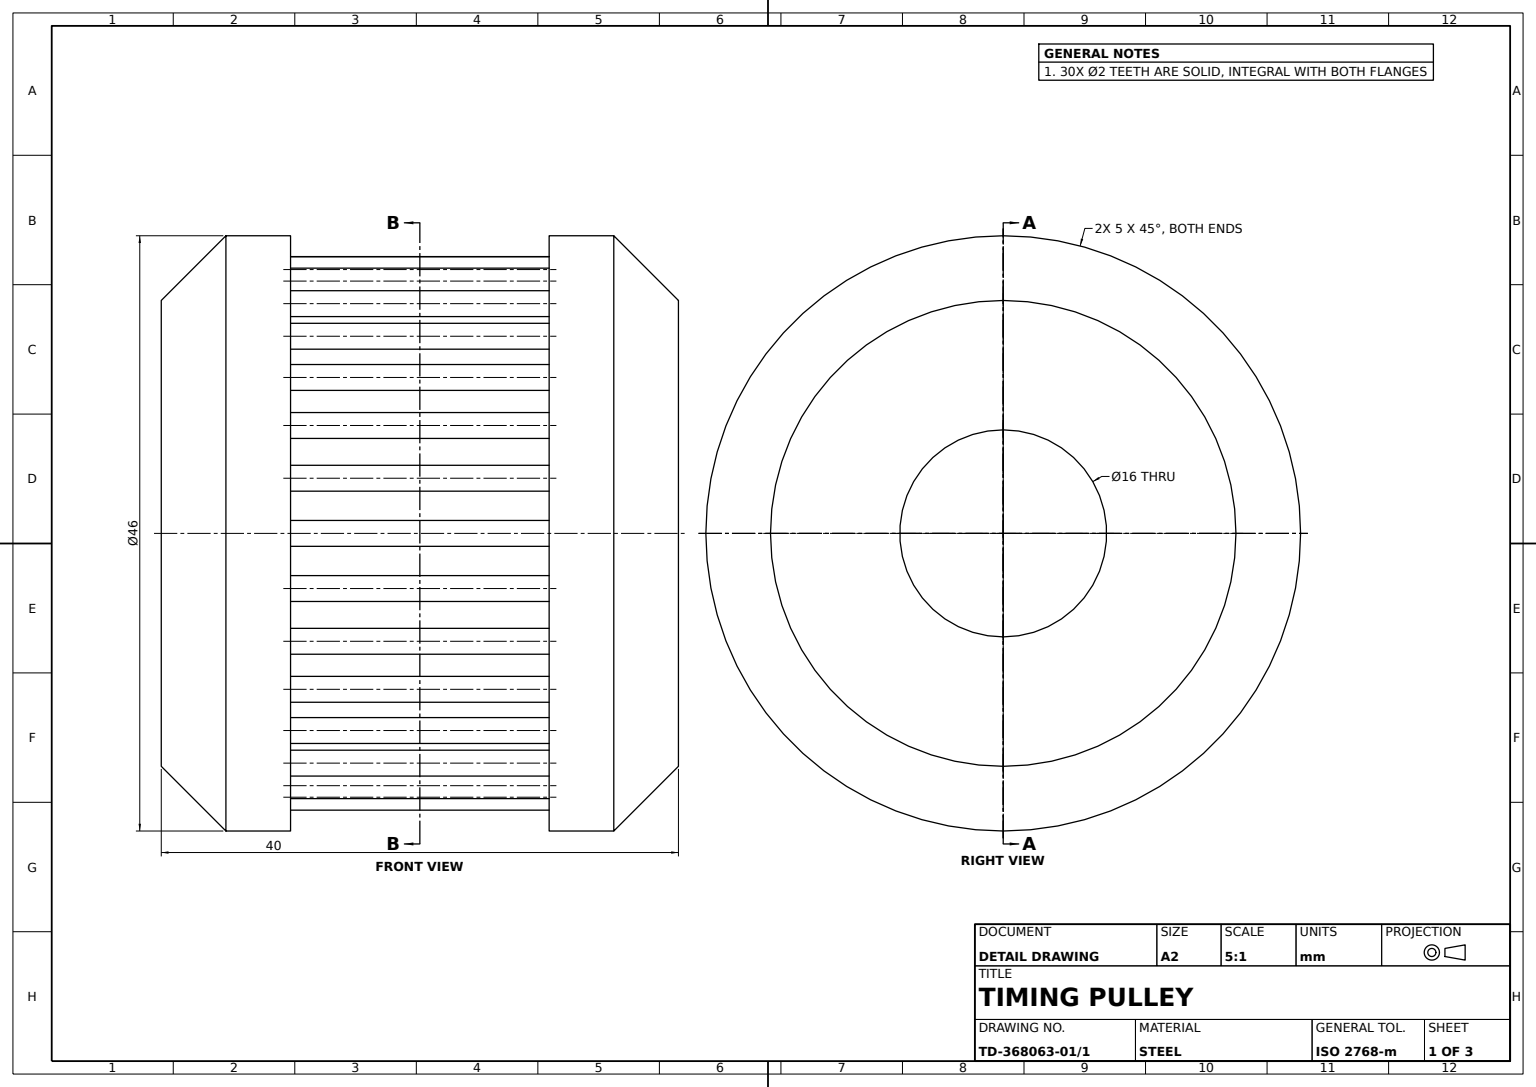
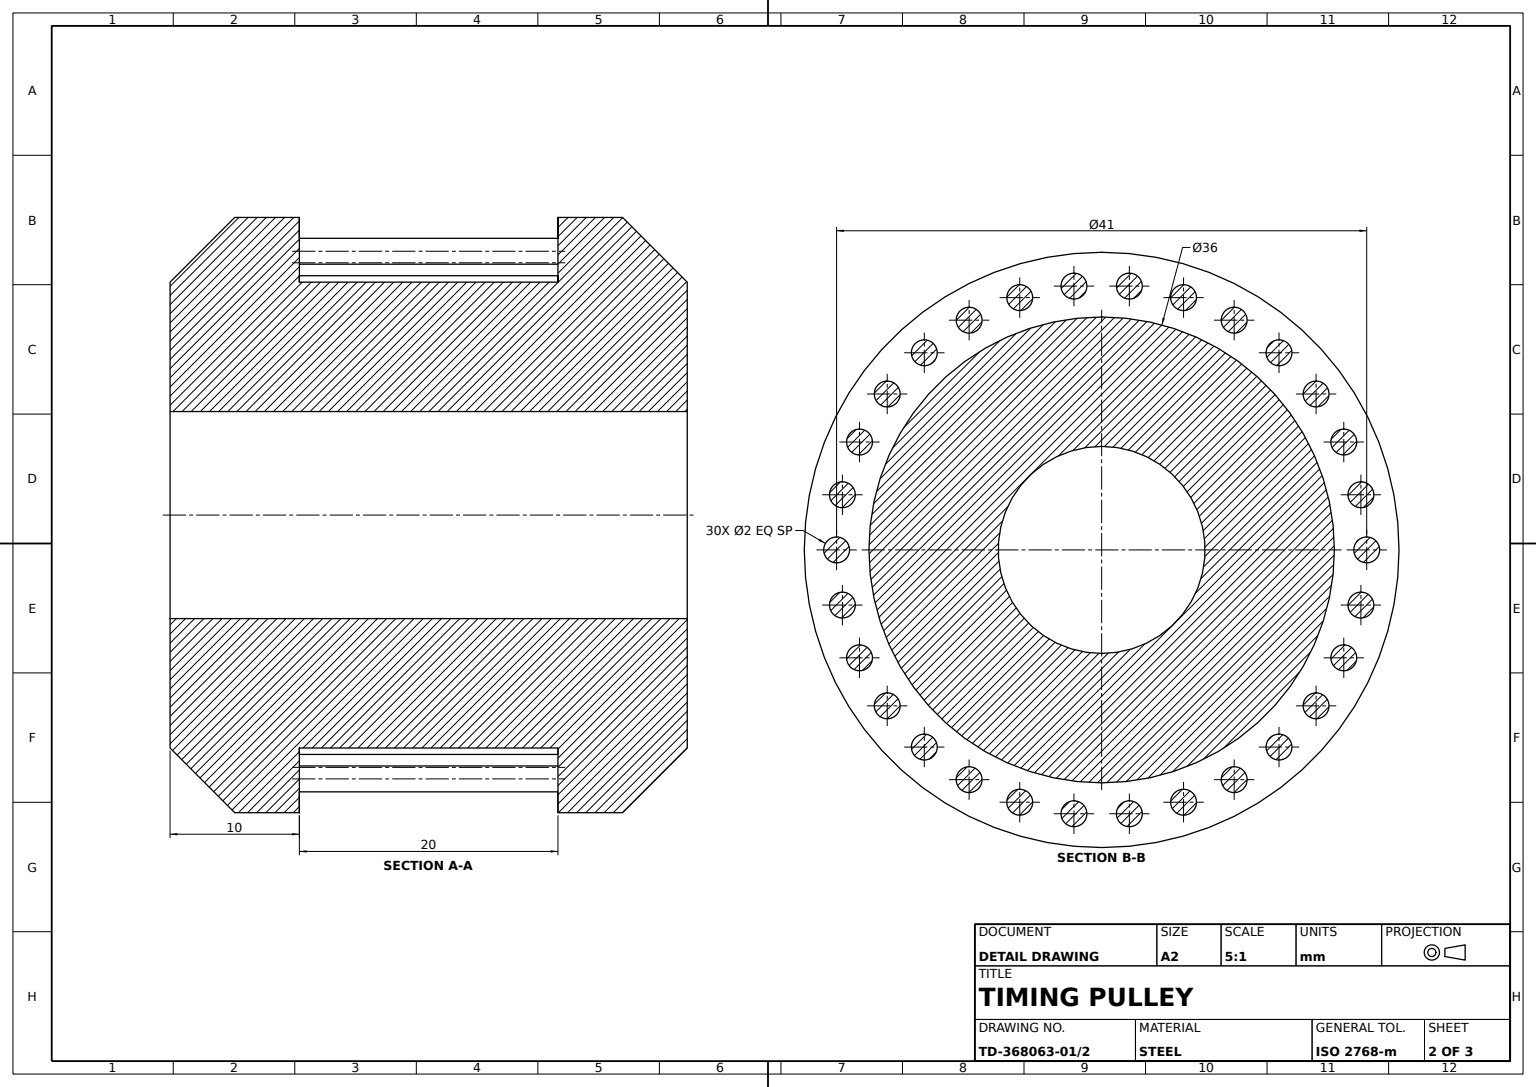
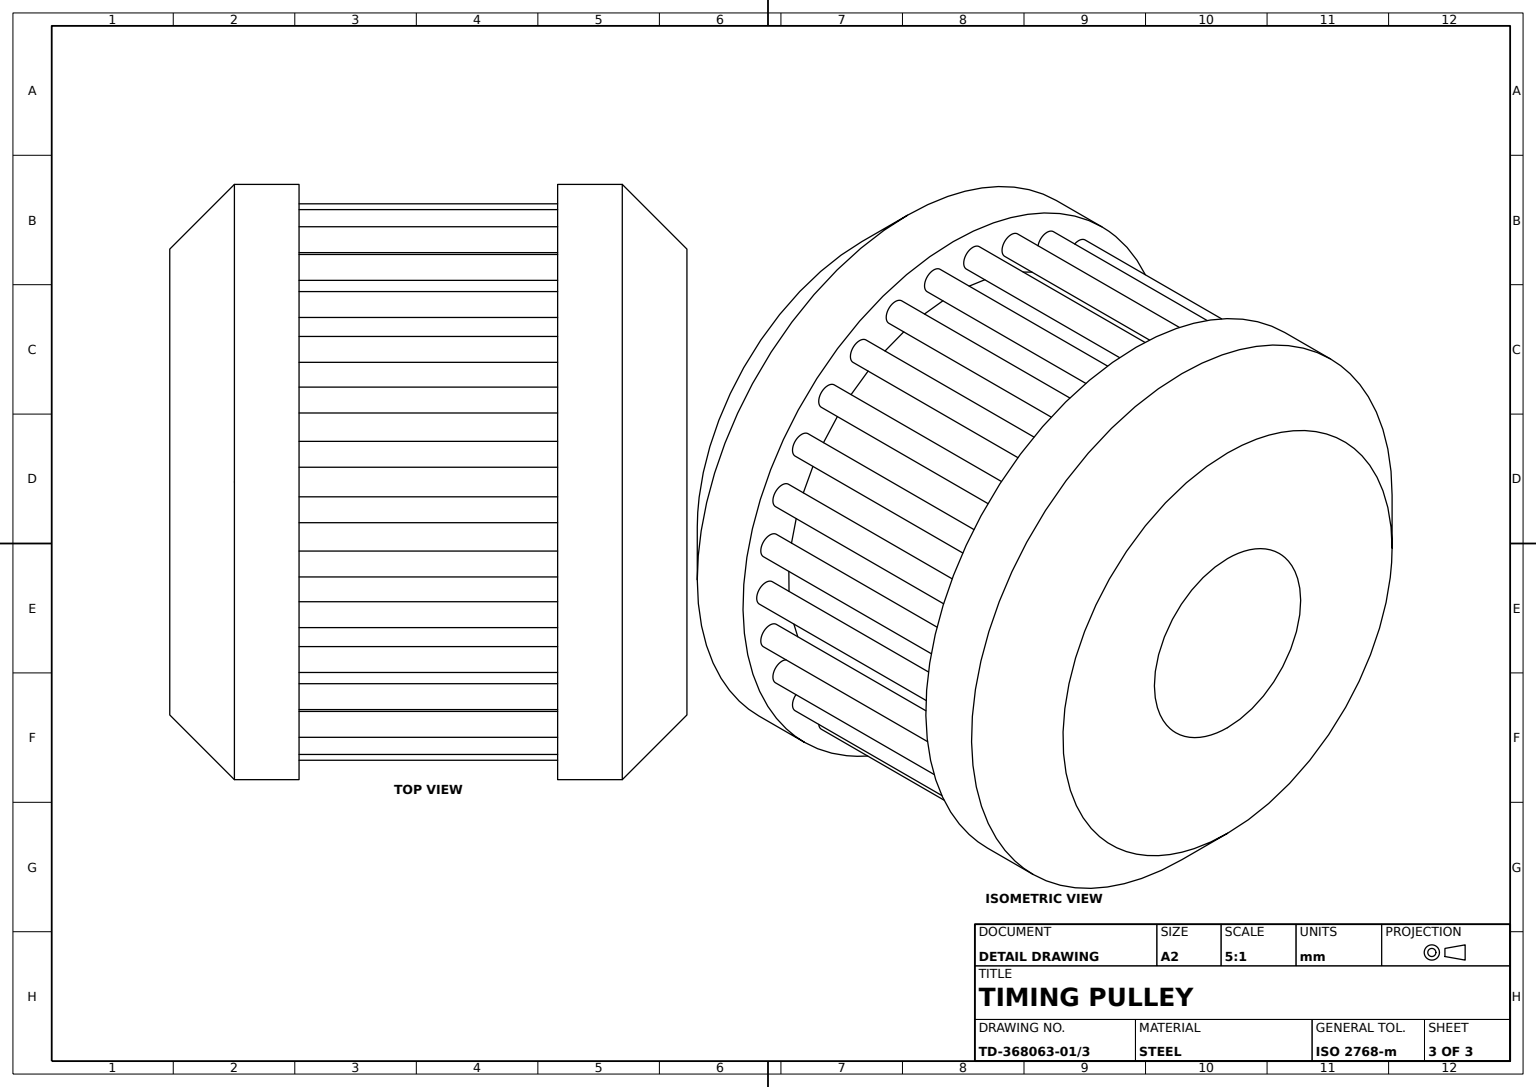
solid
v1 (-1,30,20.5)
v2 (1,30,20.5)
e1 v1 v2 CIRCLE(AX(P(0,30,20.5),D(0,-1,0),D(-1,0,0)),1)
v3 (1,10,20.5)
e2 v3 v2 LINE
v4 (-1,10,20.5)
e3 v3 v4 CIRCLE(AX(P(0,10,20.5),D(0,1,0),D(1,0,0)),1)
e4 v4 v1 LINE
face CYL(AX(P(0,10,20.5),D(0,1,0),D(-1,0,0)),1) [e1 -e2 e3 e4]
v5 (18.496659,30,-6.334848)
v6 (20.496659,30,-6.334848)
e5 v5 v6 CIRCLE(AX(P(19.496659,30,-6.334848),D(0,-1,0),D(-1,0,0)),1)
v7 (20.496659,10,-6.334848)
e6 v7 v6 LINE
v8 (18.496659,10,-6.334848)
e7 v7 v8 CIRCLE(AX(P(19.496659,10,-6.334848),D(0,1,0),D(1,0,0)),1)
e8 v8 v5 LINE
face CYL(AX(P(19.496659,10,-6.334848),D(0,1,0),D(-1,0,0)),1) [e5 -e6 e7 e8]
v9 (-18,30,0)
v10 (18,30,0)
e9 v9 v10 CIRCLE(AX(P(0,30,0),D(0,1,0),D(-1,0,0)),18)
v11 (-18,10,0)
e10 v11 v9 LINE
v12 (18,10,0)
e11 v11 v12 CIRCLE(AX(P(0,10,0),D(0,1,0),D(-1,0,0)),18)
e12 v12 v10 LINE
face CYL(AX(P(0,32.636364,0),D(0,1,0),D(-1,0,0)),18) [-e9 -e10 e11 e12]
v13 (19.387699,30,-2.142833)
v14 (21.387699,30,-2.142833)
e13 v13 v14 CIRCLE(AX(P(20.387699,30,-2.142833),D(0,-1,0),D(-1,0,0)),1)
v15 (21.387699,10,-2.142833)
e14 v15 v14 LINE
v16 (19.387699,10,-2.142833)
e15 v15 v16 CIRCLE(AX(P(20.387699,10,-2.142833),D(0,1,0),D(1,0,0)),1)
e16 v16 v13 LINE
face CYL(AX(P(20.387699,10,-2.142833),D(0,1,0),D(-1,0,0)),1) [e13 -e14 e15 e16]
v17 (23,30,0)
v18 (23,35,0)
e17 v17 v18 LINE
v19 (-23,35,0)
e18 v19 v18 CIRCLE(AX(P(0,35,0),D(0,1,0),D(-1,0,0)),23)
v20 (-23,30,0)
e19 v20 v19 LINE
e20 v20 v17 CIRCLE(AX(P(0,30,0),D(0,1,0),D(-1,0,0)),23)
face CYL(AX(P(0,32.636364,0),D(0,1,0),D(-1,0,0)),23) [e17 -e18 -e19 e20]
v21 (18,0,0)
v22 (-18,0,0)
e21 v21 v22 CIRCLE(AX(P(0,0,0),D(0,1,0),D(-1,0,0)),18)
v23 (-23,5,0)
e22 v22 v23 LINE
v24 (23,5,0)
e23 v24 v23 CIRCLE(AX(P(0,5,0),D(0,1,0),D(-1,0,0)),23)
e24 v21 v24 LINE
face CONE(AX(P(0,0,0),D(0,1,0),D(-1,0,0)),18,0.785398163) [e21 e22 -e23 -e24]
v25 (18,40,0)
e25 v25 v18 LINE
v26 (-18,40,0)
e26 v26 v25 CIRCLE(AX(P(0,40,0),D(0,1,0),D(-1,0,0)),18)
e27 v26 v19 LINE
face CONE(AX(P(0,35,0),D(0,-1,0),D(1,0,0)),23,0.785398163) [e18 -e25 -e26 e27]
v27 (-9.338101,30,18.727682)
v28 (-7.338101,30,18.727682)
e28 v27 v28 CIRCLE(AX(P(-8.338101,30,18.727682),D(0,-1,0),D(-1,0,0)),1)
v29 (-7.338101,10,18.727682)
e29 v29 v28 LINE
v30 (-9.338101,10,18.727682)
e30 v29 v30 CIRCLE(AX(P(-8.338101,10,18.727682),D(0,1,0),D(1,0,0)),1)
e31 v30 v27 LINE
face CYL(AX(P(-8.338101,10,18.727682),D(0,1,0),D(-1,0,0)),1) [e28 -e29 e30 e31]
v31 (-20.496659,10,6.334848)
v32 (-18.496659,10,6.334848)
e32 v31 v32 CIRCLE(AX(P(-19.496659,10,6.334848),D(0,1,0),D(1,0,0)),1)
v33 (-18.496659,30,6.334848)
e33 v32 v33 LINE
v34 (-20.496659,30,6.334848)
e34 v33 v34 CIRCLE(AX(P(-19.496659,30,6.334848),D(0,-1,0),D(-1,0,0)),1)
e35 v31 v34 LINE
face CYL(AX(P(-19.496659,10,6.334848),D(0,1,0),D(-1,0,0)),1) [e32 e33 e34 -e35]
v35 (14.234469,10,-13.717177)
v36 (16.234469,10,-13.717177)
e36 v35 v36 CIRCLE(AX(P(15.234469,10,-13.717177),D(0,1,0),D(1,0,0)),1)
v37 (16.234469,30,-13.717177)
e37 v36 v37 LINE
v38 (14.234469,30,-13.717177)
e38 v37 v38 CIRCLE(AX(P(15.234469,30,-13.717177),D(0,-1,0),D(-1,0,0)),1)
e39 v35 v38 LINE
face CYL(AX(P(15.234469,10,-13.717177),D(0,1,0),D(-1,0,0)),1) [e36 e37 e38 -e39]
e40 v12 v11 CIRCLE(AX(P(0,10,0),D(0,1,0),D(-1,0,0)),18)
e41 v10 v9 CIRCLE(AX(P(0,30,0),D(0,1,0),D(-1,0,0)),18)
face CYL(AX(P(0,32.636364,0),D(0,1,0),D(-1,0,0)),18) [e40 e10 -e41 -e12]
v39 (21.387699,10,2.142833)
v40 (19.387699,10,2.142833)
e42 v39 v40 CIRCLE(AX(P(20.387699,10,2.142833),D(0,1,0),D(1,0,0)),1)
v41 (19.387699,30,2.142833)
e43 v40 v41 LINE
v42 (21.387699,30,2.142833)
e44 v41 v42 CIRCLE(AX(P(20.387699,30,2.142833),D(0,-1,0),D(-1,0,0)),1)
e45 v39 v42 LINE
face CYL(AX(P(20.387699,10,2.142833),D(0,1,0),D(-1,0,0)),1) [e42 e43 e44 -e45]
v43 (20.496659,10,6.334848)
v44 (20.496659,30,6.334848)
e46 v43 v44 LINE
v45 (18.496659,10,6.334848)
e47 v43 v45 CIRCLE(AX(P(19.496659,10,6.334848),D(0,1,0),D(1,0,0)),1)
v46 (18.496659,30,6.334848)
e48 v45 v46 LINE
e49 v46 v44 CIRCLE(AX(P(19.496659,30,6.334848),D(0,-1,0),D(-1,0,0)),1)
face CYL(AX(P(19.496659,10,6.334848),D(0,1,0),D(-1,0,0)),1) [-e46 e47 e48 e49]
v47 (9.338101,10,-18.727682)
v48 (9.338101,30,-18.727682)
e50 v47 v48 LINE
v49 (7.338101,30,-18.727682)
e51 v48 v49 CIRCLE(AX(P(8.338101,30,-18.727682),D(0,-1,0),D(-1,0,0)),1)
v50 (7.338101,10,-18.727682)
e52 v50 v49 LINE
e53 v50 v47 CIRCLE(AX(P(8.338101,10,-18.727682),D(0,1,0),D(1,0,0)),1)
face CYL(AX(P(8.338101,10,-18.727682),D(0,1,0),D(-1,0,0)),1) [e50 e51 -e52 e53]
e54 v18 v19 CIRCLE(AX(P(0,35,0),D(0,1,0),D(-1,0,0)),23)
e55 v25 v26 CIRCLE(AX(P(0,40,0),D(0,1,0),D(-1,0,0)),18)
face CONE(AX(P(0,35,0),D(0,-1,0),D(1,0,0)),23,0.785398163) [e54 -e27 -e55 e25]
e56 v40 v39 CIRCLE(AX(P(20.387699,10,2.142833),D(0,1,0),D(1,0,0)),1)
e57 v42 v41 CIRCLE(AX(P(20.387699,30,2.142833),D(0,-1,0),D(-1,0,0)),1)
face CYL(AX(P(20.387699,10,2.142833),D(0,1,0),D(-1,0,0)),1) [-e43 e56 e45 e57]
v51 (-23,10,0)
e58 v23 v51 LINE
e59 v23 v24 CIRCLE(AX(P(0,5,0),D(0,1,0),D(-1,0,0)),23)
v52 (23,10,0)
e60 v24 v52 LINE
e61 v51 v52 CIRCLE(AX(P(0,10,0),D(0,1,0),D(-1,0,0)),23)
face CYL(AX(P(0,32.636364,0),D(0,1,0),D(-1,0,0)),23) [-e58 e59 e60 -e61]
e62 v32 v31 CIRCLE(AX(P(-19.496659,10,6.334848),D(0,1,0),D(1,0,0)),1)
e63 v34 v33 CIRCLE(AX(P(-19.496659,30,6.334848),D(0,-1,0),D(-1,0,0)),1)
face CYL(AX(P(-19.496659,10,6.334848),D(0,1,0),D(-1,0,0)),1) [e62 e35 e63 -e33]
v53 (-16.753521,10,10.25)
v54 (-18.753521,10,10.25)
e64 v53 v54 CIRCLE(AX(P(-17.753521,10,10.25),D(0,1,0),D(1,0,0)),1)
v55 (-18.753521,30,10.25)
e65 v54 v55 LINE
v56 (-16.753521,30,10.25)
e66 v55 v56 CIRCLE(AX(P(-17.753521,30,10.25),D(0,-1,0),D(-1,0,0)),1)
e67 v53 v56 LINE
face CYL(AX(P(-17.753521,10,10.25),D(0,1,0),D(-1,0,0)),1) [e64 e65 e66 -e67]
v57 (-19.387699,30,2.142833)
v58 (-21.387699,30,2.142833)
e68 v57 v58 CIRCLE(AX(P(-20.387699,30,2.142833),D(0,-1,0),D(-1,0,0)),1)
v59 (-21.387699,10,2.142833)
e69 v59 v58 LINE
v60 (-19.387699,10,2.142833)
e70 v59 v60 CIRCLE(AX(P(-20.387699,10,2.142833),D(0,1,0),D(1,0,0)),1)
e71 v60 v57 LINE
face CYL(AX(P(-20.387699,10,2.142833),D(0,1,0),D(-1,0,0)),1) [e68 -e69 e70 e71]
e72 v52 v51 CIRCLE(AX(P(0,10,0),D(0,1,0),D(-1,0,0)),23)
face CYL(AX(P(0,32.636364,0),D(0,1,0),D(-1,0,0)),23) [e58 -e72 -e60 e23]
v61 (5.26219,30,20.052026)
v62 (3.26219,30,20.052026)
e73 v61 v62 CIRCLE(AX(P(4.26219,30,20.052026),D(0,-1,0),D(-1,0,0)),1)
v63 (3.26219,10,20.052026)
e74 v63 v62 LINE
v64 (5.26219,10,20.052026)
e75 v63 v64 CIRCLE(AX(P(4.26219,10,20.052026),D(0,1,0),D(1,0,0)),1)
e76 v64 v61 LINE
face CYL(AX(P(4.26219,10,20.052026),D(0,1,0),D(-1,0,0)),1) [e73 -e74 e75 e76]
v65 (1,10,-20.5)
v66 (-1,10,-20.5)
e77 v65 v66 CIRCLE(AX(P(0,10,-20.5),D(0,1,0),D(1,0,0)),1)
v67 (-1,30,-20.5)
e78 v66 v67 LINE
v68 (1,30,-20.5)
e79 v67 v68 CIRCLE(AX(P(0,30,-20.5),D(0,-1,0),D(-1,0,0)),1)
e80 v65 v68 LINE
face CYL(AX(P(0,10,-20.5),D(0,1,0),D(-1,0,0)),1) [e77 e78 e79 -e80]
v69 (-8,0,0)
v70 (8,0,0)
e81 v69 v70 CIRCLE(AX(P(0,0,0),D(0,1,0),D(-1,0,0)),8)
v71 (-8,40,0)
e82 v69 v71 LINE
v72 (8,40,0)
e83 v71 v72 CIRCLE(AX(P(0,40,0),D(0,1,0),D(-1,0,0)),8)
e84 v70 v72 LINE
face CYL(AX(P(0,32.636364,0),D(0,1,0),D(-1,0,0)),8) rev [-e81 e82 e83 -e84]
v73 (18.753521,10,10.25)
v74 (18.753521,30,10.25)
e85 v73 v74 LINE
v75 (16.753521,10,10.25)
e86 v73 v75 CIRCLE(AX(P(17.753521,10,10.25),D(0,1,0),D(1,0,0)),1)
v76 (16.753521,30,10.25)
e87 v75 v76 LINE
e88 v76 v74 CIRCLE(AX(P(17.753521,30,10.25),D(0,-1,0),D(-1,0,0)),1)
face CYL(AX(P(17.753521,10,10.25),D(0,1,0),D(-1,0,0)),1) [-e85 e86 e87 e88]
v77 (13.049598,10,-16.584848)
v78 (13.049598,30,-16.584848)
e89 v77 v78 LINE
v79 (11.049598,10,-16.584848)
e90 v77 v79 CIRCLE(AX(P(12.049598,10,-16.584848),D(0,1,0),D(1,0,0)),1)
v80 (11.049598,30,-16.584848)
e91 v79 v80 LINE
e92 v80 v78 CIRCLE(AX(P(12.049598,30,-16.584848),D(0,-1,0),D(-1,0,0)),1)
face CYL(AX(P(12.049598,10,-16.584848),D(0,1,0),D(-1,0,0)),1) [-e89 e90 e91 e92]
e93 v45 v43 CIRCLE(AX(P(19.496659,10,6.334848),D(0,1,0),D(1,0,0)),1)
e94 v44 v46 CIRCLE(AX(P(19.496659,30,6.334848),D(0,-1,0),D(-1,0,0)),1)
face CYL(AX(P(19.496659,10,6.334848),D(0,1,0),D(-1,0,0)),1) [e93 e46 e94 -e48]
v81 (-16.753521,10,-10.25)
v82 (-16.753521,30,-10.25)
e95 v81 v82 LINE
v83 (-18.753521,10,-10.25)
e96 v81 v83 CIRCLE(AX(P(-17.753521,10,-10.25),D(0,1,0),D(1,0,0)),1)
v84 (-18.753521,30,-10.25)
e97 v83 v84 LINE
e98 v84 v82 CIRCLE(AX(P(-17.753521,30,-10.25),D(0,-1,0),D(-1,0,0)),1)
face CYL(AX(P(-17.753521,10,-10.25),D(0,1,0),D(-1,0,0)),1) [-e95 e96 e97 e98]
e99 v4 v3 CIRCLE(AX(P(0,10,20.5),D(0,1,0),D(1,0,0)),1)
e100 v2 v1 CIRCLE(AX(P(0,30,20.5),D(0,-1,0),D(-1,0,0)),1)
face CYL(AX(P(0,10,20.5),D(0,1,0),D(-1,0,0)),1) [-e4 e99 e2 e100]
v85 (-21.387699,10,-2.142833)
v86 (-21.387699,30,-2.142833)
e101 v85 v86 LINE
v87 (-19.387699,10,-2.142833)
e102 v85 v87 CIRCLE(AX(P(-20.387699,10,-2.142833),D(0,1,0),D(1,0,0)),1)
v88 (-19.387699,30,-2.142833)
e103 v87 v88 LINE
e104 v88 v86 CIRCLE(AX(P(-20.387699,30,-2.142833),D(0,-1,0),D(-1,0,0)),1)
face CYL(AX(P(-20.387699,10,-2.142833),D(0,1,0),D(-1,0,0)),1) [-e101 e102 e103 e104]
v89 (-5.26219,10,20.052026)
v90 (-5.26219,30,20.052026)
e105 v89 v90 LINE
v91 (-3.26219,30,20.052026)
e106 v90 v91 CIRCLE(AX(P(-4.26219,30,20.052026),D(0,-1,0),D(-1,0,0)),1)
v92 (-3.26219,10,20.052026)
e107 v92 v91 LINE
e108 v92 v89 CIRCLE(AX(P(-4.26219,10,20.052026),D(0,1,0),D(1,0,0)),1)
face CYL(AX(P(-4.26219,10,20.052026),D(0,1,0),D(-1,0,0)),1) [e105 e106 -e107 e108]
v93 (-5.26219,30,-20.052026)
v94 (-3.26219,30,-20.052026)
e109 v93 v94 CIRCLE(AX(P(-4.26219,30,-20.052026),D(0,-1,0),D(-1,0,0)),1)
e110 v94 v93 CIRCLE(AX(P(-4.26219,30,-20.052026),D(0,-1,0),D(-1,0,0)),1)
v95 (-16.234469,30,-13.717177)
v96 (-14.234469,30,-13.717177)
e111 v95 v96 CIRCLE(AX(P(-15.234469,30,-13.717177),D(0,-1,0),D(-1,0,0)),1)
e112 v96 v95 CIRCLE(AX(P(-15.234469,30,-13.717177),D(0,-1,0),D(-1,0,0)),1)
v97 (9.338101,30,18.727682)
v98 (7.338101,30,18.727682)
e113 v97 v98 CIRCLE(AX(P(8.338101,30,18.727682),D(0,-1,0),D(-1,0,0)),1)
e114 v98 v97 CIRCLE(AX(P(8.338101,30,18.727682),D(0,-1,0),D(-1,0,0)),1)
e115 v91 v90 CIRCLE(AX(P(-4.26219,30,20.052026),D(0,-1,0),D(-1,0,0)),1)
v99 (-7.338101,30,-18.727682)
v100 (-9.338101,30,-18.727682)
e116 v99 v100 CIRCLE(AX(P(-8.338101,30,-18.727682),D(0,-1,0),D(-1,0,0)),1)
e117 v100 v99 CIRCLE(AX(P(-8.338101,30,-18.727682),D(0,-1,0),D(-1,0,0)),1)
e118 v86 v88 CIRCLE(AX(P(-20.387699,30,-2.142833),D(0,-1,0),D(-1,0,0)),1)
v101 (-16.234469,30,13.717177)
v102 (-14.234469,30,13.717177)
e119 v101 v102 CIRCLE(AX(P(-15.234469,30,13.717177),D(0,-1,0),D(-1,0,0)),1)
e120 v102 v101 CIRCLE(AX(P(-15.234469,30,13.717177),D(0,-1,0),D(-1,0,0)),1)
e121 v58 v57 CIRCLE(AX(P(-20.387699,30,2.142833),D(0,-1,0),D(-1,0,0)),1)
v103 (18.753521,30,-10.25)
v104 (16.753521,30,-10.25)
e122 v103 v104 CIRCLE(AX(P(17.753521,30,-10.25),D(0,-1,0),D(-1,0,0)),1)
e123 v104 v103 CIRCLE(AX(P(17.753521,30,-10.25),D(0,-1,0),D(-1,0,0)),1)
v105 (-11.049598,30,-16.584848)
v106 (-13.049598,30,-16.584848)
e124 v105 v106 CIRCLE(AX(P(-12.049598,30,-16.584848),D(0,-1,0),D(-1,0,0)),1)
e125 v106 v105 CIRCLE(AX(P(-12.049598,30,-16.584848),D(0,-1,0),D(-1,0,0)),1)
v107 (-20.496659,30,-6.334848)
v108 (-18.496659,30,-6.334848)
e126 v107 v108 CIRCLE(AX(P(-19.496659,30,-6.334848),D(0,-1,0),D(-1,0,0)),1)
e127 v108 v107 CIRCLE(AX(P(-19.496659,30,-6.334848),D(0,-1,0),D(-1,0,0)),1)
v109 (14.234469,30,13.717177)
v110 (16.234469,30,13.717177)
e128 v109 v110 CIRCLE(AX(P(15.234469,30,13.717177),D(0,-1,0),D(-1,0,0)),1)
e129 v110 v109 CIRCLE(AX(P(15.234469,30,13.717177),D(0,-1,0),D(-1,0,0)),1)
e130 v17 v20 CIRCLE(AX(P(0,30,0),D(0,1,0),D(-1,0,0)),23)
e131 v49 v48 CIRCLE(AX(P(8.338101,30,-18.727682),D(0,-1,0),D(-1,0,0)),1)
e132 v68 v67 CIRCLE(AX(P(0,30,-20.5),D(0,-1,0),D(-1,0,0)),1)
v111 (3.26219,30,-20.052026)
v112 (5.26219,30,-20.052026)
e133 v111 v112 CIRCLE(AX(P(4.26219,30,-20.052026),D(0,-1,0),D(-1,0,0)),1)
e134 v112 v111 CIRCLE(AX(P(4.26219,30,-20.052026),D(0,-1,0),D(-1,0,0)),1)
e135 v38 v37 CIRCLE(AX(P(15.234469,30,-13.717177),D(0,-1,0),D(-1,0,0)),1)
e136 v62 v61 CIRCLE(AX(P(4.26219,30,20.052026),D(0,-1,0),D(-1,0,0)),1)
v113 (11.049598,30,16.584848)
v114 (13.049598,30,16.584848)
e137 v113 v114 CIRCLE(AX(P(12.049598,30,16.584848),D(0,-1,0),D(-1,0,0)),1)
e138 v114 v113 CIRCLE(AX(P(12.049598,30,16.584848),D(0,-1,0),D(-1,0,0)),1)
e139 v74 v76 CIRCLE(AX(P(17.753521,30,10.25),D(0,-1,0),D(-1,0,0)),1)
e140 v28 v27 CIRCLE(AX(P(-8.338101,30,18.727682),D(0,-1,0),D(-1,0,0)),1)
e141 v82 v84 CIRCLE(AX(P(-17.753521,30,-10.25),D(0,-1,0),D(-1,0,0)),1)
e142 v56 v55 CIRCLE(AX(P(-17.753521,30,10.25),D(0,-1,0),D(-1,0,0)),1)
e143 v78 v80 CIRCLE(AX(P(12.049598,30,-16.584848),D(0,-1,0),D(-1,0,0)),1)
e144 v6 v5 CIRCLE(AX(P(19.496659,30,-6.334848),D(0,-1,0),D(-1,0,0)),1)
v115 (-11.049598,30,16.584848)
v116 (-13.049598,30,16.584848)
e145 v115 v116 CIRCLE(AX(P(-12.049598,30,16.584848),D(0,-1,0),D(-1,0,0)),1)
e146 v116 v115 CIRCLE(AX(P(-12.049598,30,16.584848),D(0,-1,0),D(-1,0,0)),1)
e147 v14 v13 CIRCLE(AX(P(20.387699,30,-2.142833),D(0,-1,0),D(-1,0,0)),1)
face PLANE(AX(P(18,30,0),D(0,1,0),D(-1,0,0))) rev [-e44 -e57] [-e109 -e110] [-e111 -e112] [-e113 -e114] [-e106 -e115] [-e116 -e117] [-e118 -e104] [-e119 -e120] [-e121 -e68] [-e122 -e123] [-e124 -e125] [-e49 -e94] [-e126 -e127] [-e128 -e129] [-e20 -e130] [-e131 -e51] [e41 e9] [-e79 -e132] [-e133 -e134] [-e34 -e63] [-e38 -e135] [-e1 -e100] [-e136 -e73] [-e137 -e138] [-e139 -e88] [-e28 -e140] [-e141 -e98] [-e142 -e66] [-e143 -e92] [-e5 -e144] [-e145 -e146] [-e13 -e147]
v117 (-16.234469,10,-13.717177)
e148 v117 v95 LINE
v118 (-14.234469,10,-13.717177)
e149 v118 v96 LINE
e150 v118 v117 CIRCLE(AX(P(-15.234469,10,-13.717177),D(0,1,0),D(1,0,0)),1)
face CYL(AX(P(-15.234469,10,-13.717177),D(0,1,0),D(-1,0,0)),1) [e148 e111 -e149 e150]
v119 (16.234469,10,13.717177)
v120 (14.234469,10,13.717177)
e151 v119 v120 CIRCLE(AX(P(15.234469,10,13.717177),D(0,1,0),D(1,0,0)),1)
e152 v120 v109 LINE
e153 v119 v110 LINE
face CYL(AX(P(15.234469,10,13.717177),D(0,1,0),D(-1,0,0)),1) [e151 e152 e128 -e153]
v121 (5.26219,10,-20.052026)
v122 (3.26219,10,-20.052026)
e154 v121 v122 CIRCLE(AX(P(4.26219,10,-20.052026),D(0,1,0),D(1,0,0)),1)
e155 v122 v111 LINE
e156 v121 v112 LINE
face CYL(AX(P(4.26219,10,-20.052026),D(0,1,0),D(-1,0,0)),1) [e154 e155 e133 -e156]
v123 (-3.26219,10,-20.052026)
e157 v123 v94 LINE
v124 (-5.26219,10,-20.052026)
e158 v123 v124 CIRCLE(AX(P(-4.26219,10,-20.052026),D(0,1,0),D(1,0,0)),1)
e159 v124 v93 LINE
face CYL(AX(P(-4.26219,10,-20.052026),D(0,1,0),D(-1,0,0)),1) [e109 -e157 e158 e159]
v125 (-7.338101,10,-18.727682)
v126 (-9.338101,10,-18.727682)
e160 v125 v126 CIRCLE(AX(P(-8.338101,10,-18.727682),D(0,1,0),D(1,0,0)),1)
e161 v126 v100 LINE
e162 v125 v99 LINE
face CYL(AX(P(-8.338101,10,-18.727682),D(0,1,0),D(-1,0,0)),1) [e160 e161 e117 -e162]
e163 v72 v71 CIRCLE(AX(P(0,40,0),D(0,1,0),D(-1,0,0)),8)
face PLANE(AX(P(18,40,0),D(0,-1,0),D(1,0,0))) rev [-e83 -e163] [e55 e26]
e164 v117 v118 CIRCLE(AX(P(-15.234469,10,-13.717177),D(0,1,0),D(1,0,0)),1)
face CYL(AX(P(-15.234469,10,-13.717177),D(0,1,0),D(-1,0,0)),1) [e112 -e148 e164 e149]
e165 v66 v65 CIRCLE(AX(P(0,10,-20.5),D(0,1,0),D(1,0,0)),1)
face CYL(AX(P(0,10,-20.5),D(0,1,0),D(-1,0,0)),1) [-e78 e165 e80 e132]
v127 (-14.234469,10,13.717177)
e166 v127 v102 LINE
v128 (-16.234469,10,13.717177)
e167 v127 v128 CIRCLE(AX(P(-15.234469,10,13.717177),D(0,1,0),D(1,0,0)),1)
e168 v128 v101 LINE
face CYL(AX(P(-15.234469,10,13.717177),D(0,1,0),D(-1,0,0)),1) [e119 -e166 e167 e168]
e169 v126 v125 CIRCLE(AX(P(-8.338101,10,-18.727682),D(0,1,0),D(1,0,0)),1)
face CYL(AX(P(-8.338101,10,-18.727682),D(0,1,0),D(-1,0,0)),1) [-e161 e169 e162 e116]
v129 (7.338101,10,18.727682)
v130 (9.338101,10,18.727682)
e170 v129 v130 CIRCLE(AX(P(8.338101,10,18.727682),D(0,1,0),D(1,0,0)),1)
e171 v130 v97 LINE
e172 v129 v98 LINE
face CYL(AX(P(8.338101,10,18.727682),D(0,1,0),D(-1,0,0)),1) [e170 e171 e113 -e172]
e173 v83 v81 CIRCLE(AX(P(-17.753521,10,-10.25),D(0,1,0),D(1,0,0)),1)
face CYL(AX(P(-17.753521,10,-10.25),D(0,1,0),D(-1,0,0)),1) [-e97 e173 e95 e141]
face CYL(AX(P(0,32.636364,0),D(0,1,0),D(-1,0,0)),23) [e19 -e54 -e17 e130]
e174 v16 v15 CIRCLE(AX(P(20.387699,10,-2.142833),D(0,1,0),D(1,0,0)),1)
face CYL(AX(P(20.387699,10,-2.142833),D(0,1,0),D(-1,0,0)),1) [e14 e147 -e16 e174]
e175 v79 v77 CIRCLE(AX(P(12.049598,10,-16.584848),D(0,1,0),D(1,0,0)),1)
face CYL(AX(P(12.049598,10,-16.584848),D(0,1,0),D(-1,0,0)),1) [e143 -e91 e175 e89]
e176 v64 v63 CIRCLE(AX(P(4.26219,10,20.052026),D(0,1,0),D(1,0,0)),1)
face CYL(AX(P(4.26219,10,20.052026),D(0,1,0),D(-1,0,0)),1) [-e76 e176 e74 e136]
e177 v130 v129 CIRCLE(AX(P(8.338101,10,18.727682),D(0,1,0),D(1,0,0)),1)
face CYL(AX(P(8.338101,10,18.727682),D(0,1,0),D(-1,0,0)),1) [-e171 e177 e172 e114]
v131 (-20.496659,10,-6.334848)
e178 v131 v107 LINE
v132 (-18.496659,10,-6.334848)
e179 v132 v108 LINE
e180 v132 v131 CIRCLE(AX(P(-19.496659,10,-6.334848),D(0,1,0),D(1,0,0)),1)
face CYL(AX(P(-19.496659,10,-6.334848),D(0,1,0),D(-1,0,0)),1) [e178 e126 -e179 e180]
v133 (-11.049598,10,16.584848)
v134 (-13.049598,10,16.584848)
e181 v133 v134 CIRCLE(AX(P(-12.049598,10,16.584848),D(0,1,0),D(1,0,0)),1)
e182 v134 v116 LINE
e183 v133 v115 LINE
face CYL(AX(P(-12.049598,10,16.584848),D(0,1,0),D(-1,0,0)),1) [e181 e182 e146 -e183]
v135 (18.753521,10,-10.25)
e184 v135 v103 LINE
v136 (16.753521,10,-10.25)
e185 v135 v136 CIRCLE(AX(P(17.753521,10,-10.25),D(0,1,0),D(1,0,0)),1)
e186 v136 v104 LINE
face CYL(AX(P(17.753521,10,-10.25),D(0,1,0),D(-1,0,0)),1) [e123 -e184 e185 e186]
v137 (13.049598,10,16.584848)
e187 v137 v114 LINE
v138 (11.049598,10,16.584848)
e188 v137 v138 CIRCLE(AX(P(12.049598,10,16.584848),D(0,1,0),D(1,0,0)),1)
e189 v138 v113 LINE
face CYL(AX(P(12.049598,10,16.584848),D(0,1,0),D(-1,0,0)),1) [e137 -e187 e188 e189]
e190 v75 v73 CIRCLE(AX(P(17.753521,10,10.25),D(0,1,0),D(1,0,0)),1)
face CYL(AX(P(17.753521,10,10.25),D(0,1,0),D(-1,0,0)),1) [-e87 e190 e85 e139]
e191 v36 v35 CIRCLE(AX(P(15.234469,10,-13.717177),D(0,1,0),D(1,0,0)),1)
face CYL(AX(P(15.234469,10,-13.717177),D(0,1,0),D(-1,0,0)),1) [-e37 e191 e39 e135]
v139 (-11.049598,10,-16.584848)
e192 v139 v105 LINE
v140 (-13.049598,10,-16.584848)
e193 v139 v140 CIRCLE(AX(P(-12.049598,10,-16.584848),D(0,1,0),D(1,0,0)),1)
e194 v140 v106 LINE
face CYL(AX(P(-12.049598,10,-16.584848),D(0,1,0),D(-1,0,0)),1) [-e192 e193 e194 e125]
e195 v89 v92 CIRCLE(AX(P(-4.26219,10,20.052026),D(0,1,0),D(1,0,0)),1)
face CYL(AX(P(-4.26219,10,20.052026),D(0,1,0),D(-1,0,0)),1) [e107 e115 -e105 e195]
e196 v136 v135 CIRCLE(AX(P(17.753521,10,-10.25),D(0,1,0),D(1,0,0)),1)
face CYL(AX(P(17.753521,10,-10.25),D(0,1,0),D(-1,0,0)),1) [-e186 e196 e184 e122]
e197 v22 v21 CIRCLE(AX(P(0,0,0),D(0,1,0),D(-1,0,0)),18)
face CONE(AX(P(0,0,0),D(0,1,0),D(-1,0,0)),18,0.785398163) [e197 e24 -e59 -e22]
e198 v47 v50 CIRCLE(AX(P(8.338101,10,-18.727682),D(0,1,0),D(1,0,0)),1)
face CYL(AX(P(8.338101,10,-18.727682),D(0,1,0),D(-1,0,0)),1) [e198 e52 e131 -e50]
e199 v70 v69 CIRCLE(AX(P(0,0,0),D(0,1,0),D(-1,0,0)),8)
face CYL(AX(P(0,32.636364,0),D(0,1,0),D(-1,0,0)),8) rev [-e82 -e199 e84 e163]
face PLANE(AX(P(8,0,0),D(0,1,0),D(-1,0,0))) rev [-e197 -e21] [e199 e81]
e200 v120 v119 CIRCLE(AX(P(15.234469,10,13.717177),D(0,1,0),D(1,0,0)),1)
face CYL(AX(P(15.234469,10,13.717177),D(0,1,0),D(-1,0,0)),1) [-e152 e200 e153 e129]
e201 v124 v123 CIRCLE(AX(P(-4.26219,10,-20.052026),D(0,1,0),D(1,0,0)),1)
face CYL(AX(P(-4.26219,10,-20.052026),D(0,1,0),D(-1,0,0)),1) [e110 -e159 e201 e157]
e202 v131 v132 CIRCLE(AX(P(-19.496659,10,-6.334848),D(0,1,0),D(1,0,0)),1)
face CYL(AX(P(-19.496659,10,-6.334848),D(0,1,0),D(-1,0,0)),1) [e202 e179 e127 -e178]
e203 v122 v121 CIRCLE(AX(P(4.26219,10,-20.052026),D(0,1,0),D(1,0,0)),1)
face CYL(AX(P(4.26219,10,-20.052026),D(0,1,0),D(-1,0,0)),1) [e203 e156 e134 -e155]
e204 v30 v29 CIRCLE(AX(P(-8.338101,10,18.727682),D(0,1,0),D(1,0,0)),1)
face CYL(AX(P(-8.338101,10,18.727682),D(0,1,0),D(-1,0,0)),1) [e29 e140 -e31 e204]
e205 v128 v127 CIRCLE(AX(P(-15.234469,10,13.717177),D(0,1,0),D(1,0,0)),1)
face CYL(AX(P(-15.234469,10,13.717177),D(0,1,0),D(-1,0,0)),1) [e205 e166 e120 -e168]
e206 v8 v7 CIRCLE(AX(P(19.496659,10,-6.334848),D(0,1,0),D(1,0,0)),1)
face CYL(AX(P(19.496659,10,-6.334848),D(0,1,0),D(-1,0,0)),1) [-e8 e206 e6 e144]
e207 v138 v137 CIRCLE(AX(P(12.049598,10,16.584848),D(0,1,0),D(1,0,0)),1)
face CYL(AX(P(12.049598,10,16.584848),D(0,1,0),D(-1,0,0)),1) [e138 -e189 e207 e187]
e208 v87 v85 CIRCLE(AX(P(-20.387699,10,-2.142833),D(0,1,0),D(1,0,0)),1)
e209 v60 v59 CIRCLE(AX(P(-20.387699,10,2.142833),D(0,1,0),D(1,0,0)),1)
e210 v134 v133 CIRCLE(AX(P(-12.049598,10,16.584848),D(0,1,0),D(1,0,0)),1)
e211 v140 v139 CIRCLE(AX(P(-12.049598,10,-16.584848),D(0,1,0),D(1,0,0)),1)
e212 v54 v53 CIRCLE(AX(P(-17.753521,10,10.25),D(0,1,0),D(1,0,0)),1)
face PLANE(AX(P(23,10,0),D(0,-1,0),D(1,0,0))) rev [-e206 -e7] [-e56 -e42] [-e173 -e96] [-e86 -e190] [-e174 -e15] [-e47 -e93] [e61 e72] [-e32 -e62] [-e102 -e208] [-e70 -e209] [-e176 -e75] [-e77 -e165] [-e53 -e198] [-e154 -e203] [-e181 -e210] [-e191 -e36] [-e193 -e211] [-e3 -e99] [-e64 -e212] [-e195 -e108] [-e169 -e160] [-e11 -e40] [-e180 -e202] [-e204 -e30] [-e151 -e200] [-e188 -e207] [-e201 -e158] [-e185 -e196] [-e170 -e177] [-e164 -e150] [-e175 -e90] [-e205 -e167]
face CYL(AX(P(-20.387699,10,-2.142833),D(0,1,0),D(-1,0,0)),1) [e208 e101 e118 -e103]
face CYL(AX(P(-12.049598,10,16.584848),D(0,1,0),D(-1,0,0)),1) [e210 e183 e145 -e182]
face CYL(AX(P(-17.753521,10,10.25),D(0,1,0),D(-1,0,0)),1) [e67 e142 -e65 e212]
face CYL(AX(P(-20.387699,10,2.142833),D(0,1,0),D(-1,0,0)),1) [e69 e121 -e71 e209]
face CYL(AX(P(-12.049598,10,-16.584848),D(0,1,0),D(-1,0,0)),1) [-e194 e211 e192 e124]
